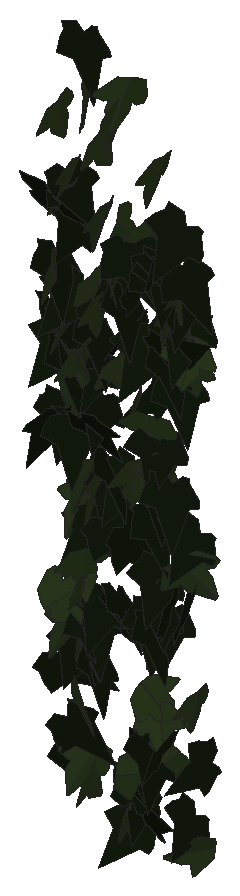
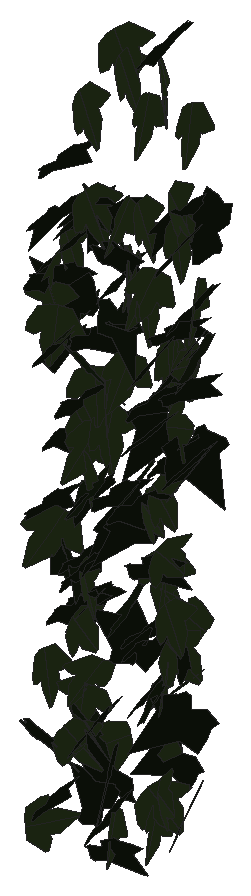
# SketchUp Ruby script. Lengths in inches.
U = 1.inch
M = Sketchup.active_model
def pt(a) = Geom::Point3d.new(a.map { |v| v * U })
def face(e, loops, mat)
  f = e.add_face(loops[0].map { |a| pt(a) })
  loops[1..].each { |l| e.add_face(l.map { |a| pt(a) }).erase! }
  f.material = f.back_material = mat if mat
  f
end
# faces: each face lists its corners as indices into pts; further lists are holes
def faces(e, pts, list, mat = nil) = list.each { |f| face(e, (f[0].is_a?(Array) ? f : [f]).map { |l| l.map { |i| pts[i] } }, mat) }
# xy, xz, yz: faces in a plane at the given z, y or x. An outline is a flat list of corners, or four numbers for a rectangle; further outlines are holes
def ring(l) = l.size == 4 ? [[l[0], l[1]], [l[2], l[1]], [l[2], l[3]], [l[0], l[3]]] : l.each_slice(2).to_a
def flat(e, list, mat, &to3) = list.each { |f| face(e, (f[0].is_a?(Array) ? f : [f]).map { |l| ring(l).map { |u, v| to3.(u, v) } }, mat) }
def xy(e, z, list, mat = nil) = flat(e, list, mat) { |x, y| [x, y, z] }
def xz(e, y, list, mat = nil) = flat(e, list, mat) { |x, z| [x, y, z] }
def yz(e, x, list, mat = nil) = flat(e, list, mat) { |y, z| [x, y, z] }
def lines(e, pts, list) = list.each { |a, b| e.add_line(pt(pts[a]), pt(pts[b])) }
# prism: a flat outline (further loops are holes) pulled along v
def prism(e, loops, v, mat = nil)
  f = face(e, loops, mat); d = Geom::Vector3d.new(v.map { |x| x * U })
  f.pushpull(f.normal.samedirection?(d) ? d.length : -d.length)
end
def box(e, o, s, mat = nil) = prism(e, [[o, [o[0] + s[0], o[1], o[2]], [o[0] + s[0], o[1] + s[1], o[2]], [o[0], o[1] + s[1], o[2]]]], [0, 0, s[2]], mat)
def at(x, y, z, deg = 0) = Geom::Transformation.translation(pt([x, y, z])) * Geom::Transformation.rotation(ORIGIN, Z_AXIS, deg.degrees)
def axes(o, x, y, z) = Geom::Transformation.new([*x, 0, *y, 0, *z, 0, *pt(o).to_a, 1])
def part(name) = M.definitions.add(name)
# library, detail: a bought-in or finely detailed component or shape, given as its bounding box
def library(name, o, s) = part(name).tap { |d| box(d.entities, o, s) }
def detail(e, o, s) = box(e.add_group.entities, o, s)
def put(e, d, t, mat = nil) = e.add_instance(d, t).tap { |i| i.material = mat if mat }
def group(e, t, mat = nil) = e.add_group.tap { |g| g.transformation = t; g.material = mat if mat }.entities
root = M.entities
M.materials.add("efeu1").color = [18, 25, 13]
M.materials.add("efeu2").color = [43, 57, 29]
c1 = part("ivyleaf_10")
p = [[0,0.5,-0.03],[-0.0625,2.02,-0.43],[-0.19,2.01,-0.46],[-0.54,1.05,-0.29],[-0.52,0.625,-0.18],[-0.83,0.76,-0.28],
  [-1.16,0.64,-0.33],[-1.15,0.33,-0.24],[-0.77,-0.39,0.02],[-0.3,-0.51,0.16],[0.04,-0.48,0.23],[-0.02,2.01,-0.4375],
  [-0.06,2.01,-0.43],[0.04,-0.49,0.23],[0.67,-0.49,0.14],[1.38,0.36,-0.2],[1.375,0.51,-0.24],[0.81,0.65,-0.19],
  [0.62,0.59,-0.15],[0.6,1.09,-0.28],[0.5,1.23,-0.31]]
faces(c1.entities,p,[[0,1,2,3,4,5,6,7,8,9,10],[11,12,0,13,14,15,16,17,18,19,20]],"efeu2")
c2 = part("ivyleaf_9")
p = [[1.54,2.16,1.25],[1.36,2.04,1.19],[-0.21,0.99,0.68],[-0.71,1.11,0.82],[-0.85,0.86,0.67],[-0.8,0.17,0.21],
  [-0.9,-0.01,0.1],[-0.67,-0.16,-0.02],[-0.08,-0.08,-0.05],[-0.03,-0.6,-0.4],[0.65,-0.88,-0.66],[0.83,-0.6,-0.49],
  [1.29,-0.42,-0.43],[1.8125,-0.07,-0.26],[1.21,0.44,0.15]]
faces(c2.entities,p,[[0,1,2,3,4,5,6,7,8,9,10,11,12,13,14]],"efeu1")
put(root,c1,axes([540.93,130.38,224.2],[-0.15644,-1.00667,-0.02735],[0.00725,0.02656,-1.01875],[1.00702,-0.15658,0.00308]))
put(root,c2,axes([542.42,130.73,223.625],[-0.06181,-0.96213,-0.06134],[0.00195,0.06134,-0.96411],[0.96408,-0.06181,-0.00198]))
put(root,c1,axes([536.875,130.09,216.64],[0.66124,0.12602,-0.83],[0.81862,0.13745,0.67305],[0.18613,-1.05226,-0.01149]))
put(root,c1,axes([540.12,130.66,241.4375],[-0.38099,-0.88498,0.32547],[-0.0074,-0.34822,-0.95549],[0.9429,-0.36032,0.12401]))
put(root,c2,axes([541.66,129.72,233.02],[-0.76894,0.3736,-0.61075],[-0.54779,0.27009,0.85489],[0.46099,0.94411,-0.00288]))
put(root,c2,axes([541.21,131.05,210.81],[0.06699,-0.97796,0.37851],[0.0144,-0.37838,-0.98019],[1.04855,0.06768,-0.01072]))
put(root,c1,axes([537.88,130.27,227.54],[-0.58914,0.23193,-0.79402],[-0.73947,0.28923,0.63314],[0.37074,0.94546,0.00109]))
put(root,c2,axes([541.61,130.62,233.7],[0.1553,-0.91969,-0.25782],[0.02046,0.26435,-0.93065],[0.95493,0.1439,0.06187]))
put(root,c2,axes([536.99,130.8,228.1875],[0.21031,-0.94092,0.02725],[-0.00073,-0.02808,-0.96411],[0.94132,0.2102,-0.00684]))
put(root,c1,axes([540.71,129.86,210.07],[-0.08364,-0.11898,-0.91944],[0.61511,0.68359,-0.14442],[0.69365,-0.62053,0.0172]))
put(root,c1,axes([538.25,130.3,240.49],[0.5345,-0.76051,-0.38517],[-0.11915,0.38351,-0.92257],[0.84412,0.53569,0.11367]))
put(root,c1,axes([537.8125,130.41,228.27],[-0.00976,-0.98445,-0.19542],[0.01306,0.19528,-0.98444],[1.00357,-0.01211,0.01091]))
put(root,c2,axes([542.66,131.17,235.54],[-0.38683,-0.82016,0.34818],[-0.06095,-0.35433,-0.90237],[0.88892,-0.38121,0.08964]))
put(root,c1,axes([538.12,130.4375,219.03],[-0.43797,-0.82794,-0.1091],[0.03624,0.10423,-0.9365],[0.83431,-0.43915,-0.01659]))
put(root,c2,axes([542.26,130.17,211.28],[-0.53623,0.78745,0.25666],[-0.16371,0.19895,-0.95242],[-0.81188,-0.56021,0.02253]))
put(root,c2,axes([536.52,130.63,224.88],[-0.06591,0.73189,-0.68623],[0.05244,-0.68426,-0.73482],[-1.00191,-0.08397,0.00668]))
put(root,c1,axes([537.0625,131.05,215.74],[-0.13106,-0.79523,0.61361],[0.03288,-0.62187,-0.79892],[1.00391,-0.08345,0.10627]))
put(root,c2,axes([539.75,131.02,231.34],[0.17196,-0.92549,0.15648],[0.016,-0.15617,-0.94125],[0.93849,0.17224,-0.01263]))
put(root,c2,axes([541.68,131.13,233.4],[0.01156,-0.96239,0.23269],[0.07273,-0.23125,-0.96005],[0.98744,0.0283,0.06799]))
put(root,c1,axes([539.7,130.8,240.47],[0.23593,-0.97411,0.15207],[0.03399,-0.14824,-1.00227],[0.98532,0.23836,-0.00184]))
put(root,c1,axes([538.06,130.55,211.29],[-0.86136,0.52009,-0.1853],[-0.15928,0.09469,1.0062],[0.52864,0.87597,0.00125]))
put(root,c1,axes([538.9375,130.33,238.8125],[0.03491,-0.87731,-0.49535],[0.0857,0.49643,-0.87319],[1.00384,-0.01187,0.09177]))
put(root,c1,axes([541.64,130.86,238.29],[0.12866,-0.99177,0.13567],[-0.00085,-0.1369,-0.99991],[1.00101,0.12736,-0.01828]))
put(root,c2,axes([540.6875,131.02,207.6875],[0.20924,-0.3432,0.85894],[0.57258,-0.64357,-0.39663],[0.72644,0.60612,0.06522]))
put(root,c1,axes([542.4,130.86,232.02],[0.2356,-0.92098,0.12448],[0.02075,-0.12317,-0.95058],[0.92912,0.23629,-0.01034]))
put(root,c2,axes([537,131.12,224.49],[-0.04574,-0.96219,0.00085],[-0.00085,-0.00081,-0.96327],[0.96219,-0.04574,-0.00081]))
put(root,c2,axes([541.57,131.16,225.36],[-0.3329,-0.87532,-0.0189],[0.00754,0.01735,-0.93649],[0.87549,-0.33298,0.00088]))
put(root,c2,axes([540.29,130.6875,234.13],[-0.08982,-0.77049,-0.6316],[0.13359,0.61912,-0.77427],[0.98728,-0.15387,0.04731]))
put(root,c1,axes([541.6,131.04,224.29],[-0.20635,-0.82514,0.38375],[-0.07608,-0.37647,-0.85041],[0.90683,-0.21935,0.01598]))
put(root,c1,axes([537.85,130.53,217.78],[0.23663,-0.82911,-0.36898],[0.0484,0.3923,-0.85048],[0.90621,0.19554,0.14176]))
put(root,c1,axes([541.28,130.74,226.18],[-0.83874,-0.38878,0.14588],[-0.12573,-0.07558,-0.92433],[0.39576,-0.84797,0.01551]))
put(root,c2,axes([535.25,130.83,234.84],[0.68573,-0.35834,0.64251],[0.5752,-0.28645,-0.77365],[0.45866,0.89498,0.00964]))
put(root,c2,axes([537.15,130.62,211.02],[-0.01913,-0.18121,-0.89416],[0.64909,0.62578,-0.1407],[0.64112,-0.63897,0.11578]))
put(root,c2,axes([536.87,131,216.28],[-0.05911,-0.05941,-1.00876],[1.00396,0.11137,-0.06539],[0.11483,-1.00434,0.05242]))
put(root,c1,axes([536.56,130.6,239.34],[-0.01158,-0.92088,-0.36017],[0.07275,0.35843,-0.91875],[0.98613,-0.03725,0.06355]))
put(root,c2,axes([538.06,130.42,225.32],[0.9375,0.21083,-0.15179],[-0.15051,-0.0225,-0.96085],[-0.21175,0.94944,0.01094]))
put(root,c1,axes([536.27,130.53,231.67],[0.32554,-0.81031,-0.47547],[0.05872,0.51977,-0.8456],[0.93767,0.24877,0.21803]))
put(root,c2,axes([536.91,131.47,214.09],[-0.1831,-0.76964,0.39862],[0.12479,-0.42659,-0.76631],[0.85772,-0.10223,0.19659]))
put(root,c2,axes([541.73,131.33,228.79],[0.19368,-0.85237,0.3665],[0.25104,-0.31229,-0.85897],[0.89322,0.2726,0.16194]))
put(root,c1,axes([537.67,131.23,222.54],[0.10183,-0.85814,0.37338],[0.08227,-0.36593,-0.86343],[0.93223,0.12603,0.03542]))
put(root,c2,axes([540.48,130.66,208.49],[-0.67854,0.37308,0.5768],[0.47051,-0.33831,0.77232],[0.50052,0.82381,0.05594]))
put(root,c2,axes([538.03,131.19,215.93],[-0.06166,-0.91246,-0.19558],[0.04429,0.19293,-0.91403],[0.93213,-0.06953,0.03049]))
put(root,c2,axes([537.38,131.3,242.61],[0.17491,-0.98607,0.00592],[0.02039,-0.0024,-1.00126],[0.98587,0.17499,0.01965]))
put(root,c2,axes([541.04,131.25,216.5],[0.22982,-0.87455,0.01617],[0.0044,-0.01557,-0.90425],[0.87469,0.22987,0.0003]))
put(root,c1,axes([538.51,130.91,230.85],[0.08623,-0.95502,-0.15053],[0.01489,0.15242,-0.95849],[0.9667,0.08284,0.02819]))
put(root,c1,axes([536.8,130.3,228.2],[0.20576,-0.34128,0.92237],[-0.43595,0.81305,0.39808],[-0.88158,-0.48172,0.01843]))
put(root,c2,axes([538.04,131.37,213.8125],[0.21086,-0.8507,0.15451],[0.00667,-0.15743,-0.8759],[0.86459,0.20869,-0.03093]))
put(root,c2,axes([543.29,130.24,217.72],[-0.02107,0.40421,0.86753],[-0.0843,0.86358,-0.40442],[-0.95335,-0.08529,0.01659]))
put(root,c2,axes([538.2,131.57,216.48],[-0.24166,-0.83129,0.24224],[0.04387,-0.26293,-0.85853],[0.86476,-0.21897,0.11125]))
put(root,c1,axes([537.67,131.46,209.26],[-0.46755,-0.68496,0.55005],[-0.10888,-0.57311,-0.80624],[0.8717,-0.43898,0.19432]))
put(root,c2,axes([541.17,131.625,218.8],[-0.25229,-0.85266,0.19023],[0.03892,-0.20878,-0.88418],[0.87276,-0.23717,0.09442]))
put(root,c1,axes([541.42,131.04,212.48],[0.86398,0.29336,0.24652],[0.22753,0.09651,-0.91225],[-0.30833,0.89326,0.0176]))
put(root,c2,axes([541.71,131.18,229.24],[0.02817,-0.10496,0.97462],[0.84911,-0.48457,-0.07673],[0.4898,0.84609,0.07696]))
put(root,c1,axes([537.93,131.5625,221.94],[0.36474,-0.7031,0.53576],[0.25972,-0.46875,-0.79198],[0.84494,0.4476,0.01217]))
put(root,c2,axes([536.59,131.85,233.65],[-0.13925,-0.75943,0.57512],[-0.01814,-0.57901,-0.76896],[0.95245,-0.12206,0.06944]))
put(root,c2,axes([536.3,131.78,229.01],[0.03651,-0.83414,0.48184],[0.04458,-0.4802,-0.83469],[0.96228,0.0539,0.02039]))
put(root,c2,axes([541,131.49,216.97],[-0.24425,-0.86165,-0.14163],[0.02837,0.13916,-0.89554],[0.87275,-0.24566,-0.01052]))
put(root,c2,axes([539.08,131.35,217.11],[0.49486,-0.7498,0.06909],[0.04077,-0.05587,-0.89837],[0.75187,0.49653,0.00325]))
put(root,c2,axes([536.15,131.84,227.91],[-0.52796,-0.72287,0.34937],[-0.10522,-0.35224,-0.88781],[0.79595,-0.52605,0.11438]))
put(root,c2,axes([540.9,131.34,221.51],[0.22205,-0.8651,-0.19712],[-0.06249,0.18744,-0.89304],[0.88507,0.23027,-0.0136]))
put(root,c1,axes([541.84,131.44,210.52],[-0.46694,-0.4314,0.62761],[-0.45846,-0.42862,-0.63572],[0.60813,-0.65438,0.00264]))
put(root,c2,axes([536.72,131.85,230.3],[-0.58843,-0.66178,0.34522],[-0.09461,-0.36992,-0.8704],[0.74039,-0.57323,0.16314]))
put(root,c2,axes([535.75,131.61,231.625],[0.1615,-0.95761,0.10475],[0.00526,-0.10534,-0.97106],[0.96331,0.16112,-0.01226]))
put(root,c2,axes([538.94,130.87,220.74],[0.18386,-0.51268,-0.7806],[0.04393,0.79945,-0.51472],[0.93287,0.0634,0.17809]))
put(root,c2,axes([539.95,130.78,220.71],[0.33511,-0.48439,-0.83189],[-0.3995,0.73144,-0.58683],[0.87583,0.51897,0.05062]))
put(root,c1,axes([539.03,131.03,231.97],[-0.50601,0.80714,0.03517],[-0.00925,0.03571,-0.95257],[-0.80785,-0.50598,-0.01112]))
put(root,c1,axes([541.09,130.82,213.53],[0.28127,0.73337,0.51824],[0.20158,0.47764,-0.78532],[-0.87508,0.34575,-0.01433]))
put(root,c2,axes([535.92,131.84,224.58],[-0.04059,-0.89422,0.31066],[0.06735,-0.31289,-0.89182],[0.94424,-0.01612,0.07697]))
put(root,c1,axes([538.3125,131.43,234.75],[0.22051,-0.95136,0.0916],[0.00913,-0.0919,-0.97651],[0.95572,0.22038,-0.0118]))
put(root,c1,axes([537.24,130.82,225.53],[-0.2868,0.26981,-0.92976],[-0.68756,0.62591,0.39372],[0.68156,0.74495,0.00594]))
put(root,c2,axes([535.55,131.53,229.32],[0.52819,-0.79931,0.11524],[0.04994,-0.1051,-0.95792],[0.80602,0.5303,-0.01616]))
put(root,c1,axes([536.5,131.64,236.03],[0.33413,-0.86401,0.32754],[0.08688,-0.31738,-0.92583],[0.91992,0.3438,-0.03153]))
put(root,c2,axes([542.03,131.875,232.02],[-0.05418,-0.91368,0.2806],[0.06798,-0.28402,-0.91169],[0.95337,-0.03167,0.08095]))
put(root,c2,axes([542.52,131.33,233.5],[0.27015,-0.85523,-0.40836],[-0.01455,0.42083,-0.89098],[0.94761,0.25028,0.10274]))
put(root,c1,axes([541.38,131.22,222.73],[0.70119,-0.53462,-0.30281],[-0.16315,0.28097,-0.87385],[0.59237,0.71022,0.11776]))
put(root,c1,axes([542.76,131.45,229.87],[0.93315,0.17375,-0.09025],[-0.08579,-0.03221,-0.94905],[-0.176,0.93695,-0.01589]))
put(root,c2,axes([536.125,132.04,208.4375],[-0.18567,-0.17571,0.87269],[-0.08884,-0.88336,-0.19676],[0.88575,-0.12544,0.1632]))
put(root,c2,axes([538.41,131.73,222.91],[0.34288,-0.84782,0.1484],[0.05281,-0.13872,-0.91452],[0.85909,0.34691,-0.00301]))
put(root,c1,axes([541.17,130.96,223.74],[-0.32173,-0.71471,-0.68752],[0.35357,0.59264,-0.78152],[0.92655,-0.47432,0.05949]))
put(root,c1,axes([543.18,131.92,206.4],[-0.17804,0.12447,-0.83945],[-0.59958,-0.62545,0.03443],[-0.60056,0.58752,0.21449]))
put(root,c1,axes([538.18,131.05,231.65],[-0.34268,-0.71439,-0.57467],[0.26903,0.50815,-0.79211],[0.87648,-0.43528,0.01845]))
put(root,c2,axes([539.8,131.1,229.73],[-0.3221,0.88597,-0.01251],[0.00687,-0.01081,-0.9427],[-0.88603,-0.32216,-0.00276]))
put(root,c2,axes([542.29,130.8,217.87],[-0.46667,0.23696,-0.90256],[-0.83819,0.33707,0.52188],[0.41012,0.95852,0.0396]))
put(root,c1,axes([540.71,131.69,234.59],[-0.21896,-0.903,0.26053],[-0.05045,-0.25583,-0.9291],[0.93847,-0.22444,0.01084]))
put(root,c2,axes([542.05,131.76,227.9],[0.02745,-0.93901,-0.13122],[0.01561,0.1317,-0.93921],[0.948,0.02502,0.01927]))
put(root,c2,axes([542.45,131.88,230.86],[-0.50733,-0.8205,-0.11291],[0.0459,0.10435,-0.96455],[0.82696,-0.50916,-0.01573]))
put(root,c2,axes([540.35,132.02,228.99],[-0.58877,-0.74701,0.11521],[-0.03968,-0.11529,-0.95031],[0.7548,-0.58876,0.03991]))
put(root,c2,axes([537.68,132.08,225.5],[-0.11719,-0.88757,0.32642],[0.10036,-0.33873,-0.88502],[0.94035,-0.07447,0.13513]))
put(root,c2,axes([539.75,131.78,232.79],[-0.9413,-0.1632,0.03486],[-0.03769,0.01332,-0.95514],[0.16257,-0.94185,-0.01955]))
put(root,c2,axes([537.75,131.96,219.73],[-0.7385,-0.51051,0.1413],[-0.10416,-0.09774,-0.89753],[0.51936,-0.74552,0.02091]))
put(root,c2,axes([541.56,131.57,227.5625],[-0.85123,0.40612,0.03095],[-0.07249,-0.08051,-0.93741],[-0.4008,-0.84797,0.10382]))
put(root,c2,axes([538.59,131.66,215.84],[0.28688,-0.24385,0.81417],[0.6592,-0.47854,-0.37561],[0.53645,0.71844,0.02616]))
put(root,c2,axes([542.4375,132.12,207.66],[-0.17823,-0.72956,0.40766],[-0.05874,-0.40486,-0.75023],[0.83367,-0.1845,0.03429]))
put(root,c2,axes([542.61,132.15,220.81],[-0.35353,-0.77644,0.33534],[-0.07165,-0.33466,-0.85039],[0.84272,-0.35418,0.06837]))
put(root,c1,axes([539.1,131.31,232.49],[0.45919,-0.77091,-0.40072],[-0.06678,0.42059,-0.88565],[0.86627,0.44106,0.14414]))
put(root,c1,axes([536.77,131.71,217.74],[-0.05337,-0.87974,0.16389],[-0.0172,-0.16315,-0.88133],[0.89472,-0.05562,-0.00716]))
put(root,c2,axes([539.8,131.92,206.52],[-0.73962,-0.3966,0.09658],[-0.08963,-0.03722,-0.83919],[0.39823,-0.74497,-0.00949]))
put(root,c2,axes([540.53,132.1,221.75],[0.12734,-0.75514,0.53029],[0.22669,-0.49331,-0.75691],[0.89446,0.23253,0.11634]))
put(root,c2,axes([535.66,131.78,224.51],[0.39219,-0.87273,-0.02052],[-0.00904,0.01844,-0.9568],[0.87293,0.39229,-0.00069]))
put(root,c2,axes([537.43,131.95,228.83],[0.25794,-0.92257,0.11035],[0.02663,-0.10714,-0.95795],[0.92877,0.25929,-0.00318]))
put(root,c1,axes([539.79,131.25,207.45],[0.2315,-0.74472,-0.50283],[0.00798,0.52094,-0.76786],[0.89854,0.18724,0.13637]))
put(root,c1,axes([542.93,131.58,213.56],[-0.02081,-0.91207,-0.09024],[-0.00791,0.09044,-0.91225],[0.91649,-0.01993,-0.00992]))
put(root,c1,axes([537.76,131.24,208.29],[0.08095,-0.74044,-0.52048],[0.03167,0.52455,-0.74131],[0.90451,0.0479,0.07254]))
put(root,c2,axes([537.26,132.17,213.86],[0.15237,-0.6407,0.59543],[0.12493,-0.58226,-0.6585],[0.8657,0.1968,-0.00977]))
put(root,c1,axes([537.23,131.26,214.98],[0.36409,-0.63901,-0.50636],[-0.01092,0.55068,-0.7028],[0.81524,0.29276,0.21672]))
put(root,c2,axes([541.25,132.04,216.76],[-0.25126,-0.88041,-0.04633],[0.0115,0.0449,-0.91556],[0.88156,-0.25152,-0.00126]))
put(root,c1,axes([540.94,132.09,216.03],[-0.05489,-0.73977,0.53334],[0.1636,-0.53362,-0.72333],[0.89719,0.05205,0.16453]))
put(root,c2,axes([536.33,131.63,235.67],[0.25319,-0.84427,-0.44731],[-0.07722,0.44315,-0.88014],[0.95232,0.2604,0.04756]))
put(root,c2,axes([537.38,132.23,227.14],[-0.26976,-0.86744,0.2219],[-0.01489,-0.22738,-0.90694],[0.89525,-0.26516,0.05178]))
put(root,c2,axes([539.6,132.25,207.92],[0.03683,-0.86836,0.3748],[-0.02165,-0.37576,-0.86845],[0.94554,0.02522,-0.03448]))
put(root,c1,axes([540.88,131.76,218.12],[0.34092,-0.83939,-0.00188],[0.00443,0.00383,-0.90596],[0.83938,0.3409,0.00555]))
put(root,c2,axes([539.18,132.28,222.48],[-0.45032,-0.76995,0.24056],[-0.07515,-0.23427,-0.89048],[0.80315,-0.45362,0.05156]))
put(root,c1,axes([539.3,131.19,234.5],[0.17729,-0.68183,-0.69468],[0.16068,0.71692,-0.66265],[0.96003,0.00593,0.2392]))
put(root,c1,axes([536.63,132.28,220.63],[-0.23085,-0.65604,0.68278],[0.25638,-0.71984,-0.60496],[0.91151,0.03632,0.34308]))
put(root,c2,axes([540.74,132.33,218.59],[-0.18593,-0.84422,0.35375],[-0.0532,-0.3504,-0.86418],[0.91379,-0.19218,0.02166]))
put(root,c1,axes([542.24,131.64,231.83],[-0.27154,0.903,-0.16027],[0.07823,-0.14373,-0.94237],[-0.91377,-0.28064,-0.03305]))
put(root,c1,axes([542.59,131.375,219.67],[-0.68827,-0.54516,-0.57548],[0.45828,0.3482,-0.87796],[0.6468,-0.82683,0.0097]))
put(root,c1,axes([536.71,132.19,209.9],[0.34336,-0.58295,0.65261],[0.40566,-0.51513,-0.67358],[0.77535,0.52767,0.0634]))
put(root,c2,axes([536.25,131.19,213.44],[-0.02043,-0.10693,-0.99921],[0.25037,0.96736,-0.10864],[0.97322,-0.2511,0.00698]))
put(root,c2,axes([538.2,132.15,222.29],[-0.26184,-0.87659,-0.0428],[0.01414,0.04044,-0.91485],[0.87752,-0.26221,0.00197]))
put(root,c1,axes([539.96,131.56,226.67],[0.35307,-0.79138,-0.35145],[-0.04157,0.36362,-0.86053],[0.86491,0.34052,0.10211]))
put(root,c1,axes([536.34,131.75,234.85],[0.02619,-0.97942,-0.10575],[0.00617,0.10595,-0.97973],[0.98509,0.02538,0.00895]))
put(root,c2,axes([543.41,131.9,210.55],[-0.84641,0.15478,0.08343],[-0.08474,0.00032,-0.86031],[-0.15406,-0.85051,0.01485]))
put(root,c2,axes([539.83,131.34,210.28],[0.3945,-0.20496,-0.81986],[-0.72596,0.381,-0.44457],[0.43263,0.82622,0.00162]))
put(root,c1,axes([539.04,131.47,227.85],[-0.33985,-0.76653,-0.47902],[0.21717,0.42753,-0.83821],[0.87742,-0.40271,0.02193]))
put(root,c1,axes([542.44,131.67,228.88],[-0.91538,-0.25601,0.01241],[-0.01915,0.02243,-0.95013],[0.2556,-0.91519,-0.02676]))
